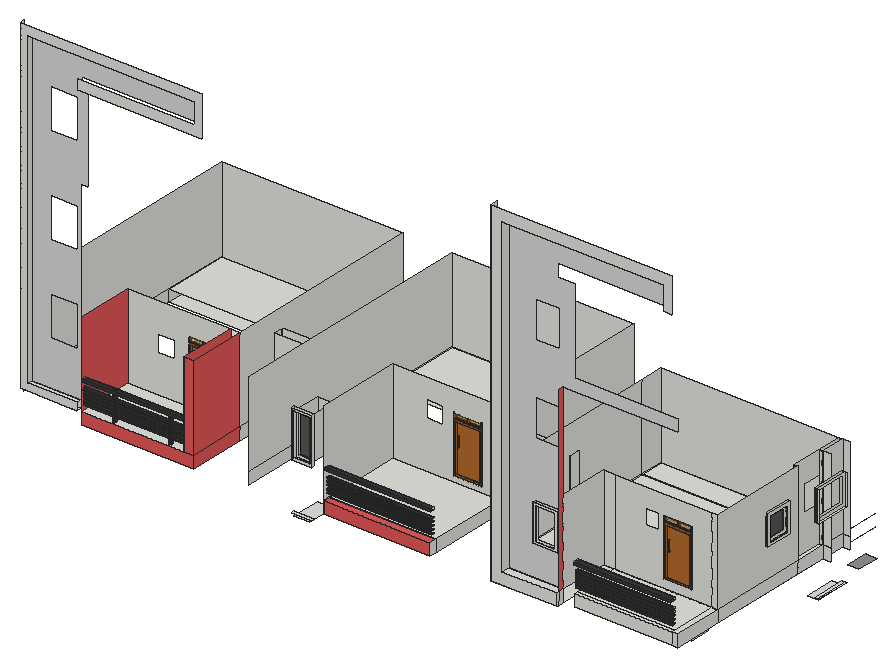
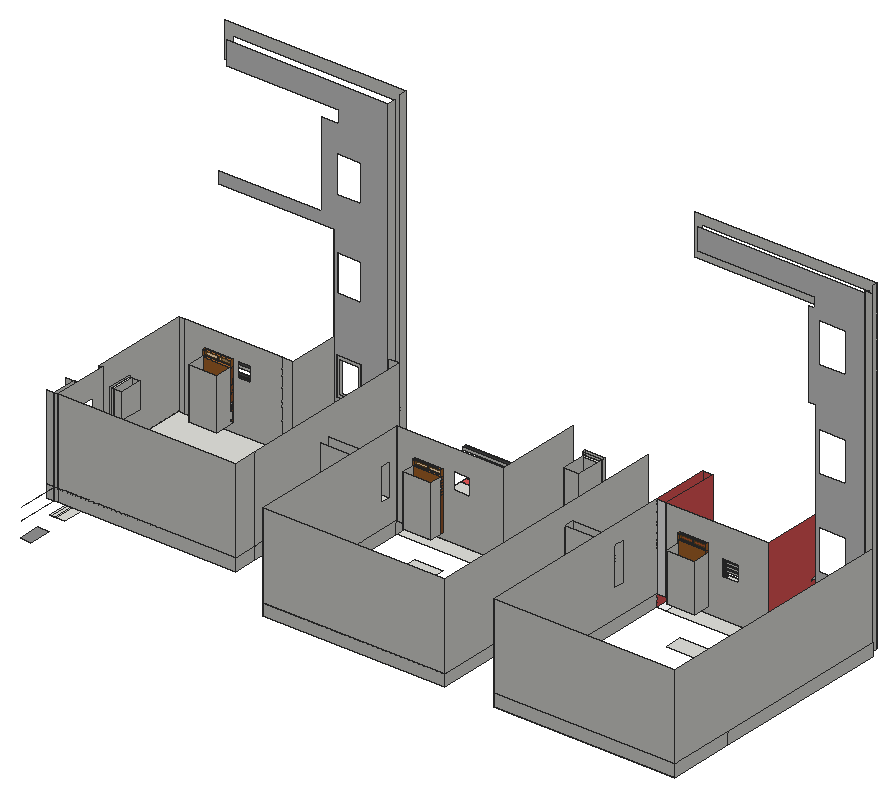
# SketchUp Ruby script. Lengths in inches.
U = 1.inch
M = Sketchup.active_model
def pt(a) = Geom::Point3d.new(a.map { |v| v * U })
def face(e, loops, mat)
  f = e.add_face(loops[0].map { |a| pt(a) })
  loops[1..].each { |l| e.add_face(l.map { |a| pt(a) }).erase! }
  f.material = f.back_material = mat if mat
  f
end
# faces: each face lists its corners as indices into pts; further lists are holes
def faces(e, pts, list, mat = nil) = list.each { |f| face(e, (f[0].is_a?(Array) ? f : [f]).map { |l| l.map { |i| pts[i] } }, mat) }
# xy, xz, yz: faces in a plane at the given z, y or x. An outline is a flat list of corners, or four numbers for a rectangle; further outlines are holes
def ring(l) = l.size == 4 ? [[l[0], l[1]], [l[2], l[1]], [l[2], l[3]], [l[0], l[3]]] : l.each_slice(2).to_a
def flat(e, list, mat, &to3) = list.each { |f| face(e, (f[0].is_a?(Array) ? f : [f]).map { |l| ring(l).map { |u, v| to3.(u, v) } }, mat) }
def xy(e, z, list, mat = nil) = flat(e, list, mat) { |x, y| [x, y, z] }
def xz(e, y, list, mat = nil) = flat(e, list, mat) { |x, z| [x, y, z] }
def yz(e, x, list, mat = nil) = flat(e, list, mat) { |y, z| [x, y, z] }
def lines(e, pts, list) = list.each { |a, b| e.add_line(pt(pts[a]), pt(pts[b])) }
# prism: a flat outline (further loops are holes) pulled along v
def prism(e, loops, v, mat = nil)
  f = face(e, loops, mat); d = Geom::Vector3d.new(v.map { |x| x * U })
  f.pushpull(f.normal.samedirection?(d) ? d.length : -d.length)
end
def box(e, o, s, mat = nil) = prism(e, [[o, [o[0] + s[0], o[1], o[2]], [o[0] + s[0], o[1] + s[1], o[2]], [o[0], o[1] + s[1], o[2]]]], [0, 0, s[2]], mat)
def at(x, y, z, deg = 0) = Geom::Transformation.translation(pt([x, y, z])) * Geom::Transformation.rotation(ORIGIN, Z_AXIS, deg.degrees)
def axes(o, x, y, z) = Geom::Transformation.new([*x, 0, *y, 0, *z, 0, *pt(o).to_a, 1])
def part(name) = M.definitions.add(name)
# library, detail: a bought-in or finely detailed component or shape, given as its bounding box
def library(name, o, s) = part(name).tap { |d| box(d.entities, o, s) }
def detail(e, o, s) = box(e.add_group.entities, o, s)
def put(e, d, t, mat = nil) = e.add_instance(d, t).tap { |i| i.material = mat if mat }
def group(e, t, mat = nil) = e.add_group.tap { |g| g.transformation = t; g.material = mat if mat }.entities
root = M.entities
M.materials.add("Generic").color = [145, 145, 145]
M.materials.add("Generic\#2").color = [229, 87, 87]
M.materials.add("Generic\#3").color = [216, 216, 216]
M.materials.add("[Color M00]").color = [255, 255, 255]
M.materials.add("[Color M07]").color = [58, 58, 58]
M.materials.add("[Color M08]").color = [45, 45, 45]
M.materials.add("[Translucent Glass Dark Green]").color = [168, 100, 12]
M.materials["[Translucent Glass Dark Green]"].alpha = 0.5
M.materials.add("[Translucent Glass Gray]").color = [0, 0, 0]
M.materials["[Translucent Glass Gray]"].alpha = 0.62
M.materials.add("[Wood Bamboo]").color = [177, 105, 43]
M.materials.add("[Wood Cherry Original]").color = [152, 86, 42]
c1 = part("Group\#10")
xy(c1.entities,0,[[0,1.08,55.8125,6.01]],"[Wood Cherry Original]")
xy(c1.entities,3.96,[[3.96,1.08,51.86,3.01]],"[Wood Bamboo]")
xy(c1.entities,51.66,[[8.63,0,9.88,3.01]],"[Color M08]")
xy(c1.entities,52.54,[[8.63,0.6875,9.88,3.01]],"[Color M08]")
xy(c1.entities,71.82,[[8.63,0.6875,9.88,3.01]],"[Color M08]")
xy(c1.entities,72.69,[[8.63,0,9.88,3.01]],"[Color M08]")
xy(c1.entities,97.36,[[3.96,1.08,51.86,3.01]],"[Wood Bamboo]")
xy(c1.entities,101.3125,[[0,1.08,55.8125,6.01]],"[Wood Bamboo]")
xy(c1.entities,102.55,[[1.23,1.08,27.29,3.01],[27.29,1.08,28.52,1.95],[28.52,1.08,54.58,3.01]],"[Wood Bamboo]")
xy(c1.entities,112.31,[[1.23,1.08,1.23,3.01,27.29,3.01,27.29,1.95,28.52,1.95,28.52,3.01,54.58,3.01,54.58,1.08]],"[Wood Bamboo]")
xy(c1.entities,113.54,[[0,1.08,55.8125,6.01]],"[Wood Bamboo]")
xz(c1.entities,0,[[8.63,51.66,9.88,72.69]],"[Color M08]")
xz(c1.entities,0.6875,[[8.63,52.54,9.88,71.82]])
xz(c1.entities,1.08,[[0,101.3125,55.8125,102.55],[0,102.55,1.23,102.55,1.23,112.31,54.58,112.31,54.58,102.55,55.8125,102.55,55.8125,113.54,0,113.54]],"[Wood Bamboo]")
xz(c1.entities,1.08,[[[0,0,55.8125,101.3125],[3.96,3.96,51.86,97.36]]],"[Wood Cherry Original]")
xz(c1.entities,1.95,[[27.29,102.55,28.52,112.31]],"[Wood Bamboo]")
xz(c1.entities,3.01,[[8.63,71.82,9.88,72.69]])
xz(c1.entities,3.01,[[1.23,102.55,27.29,112.31],[28.52,102.55,54.58,112.31]],"[Translucent Glass Dark Green]")
xz(c1.entities,3.01,[[[3.96,3.96,51.86,97.36],[8.63,71.82,9.88,72.69],[8.63,51.66,9.88,52.54]]],"[Wood Bamboo]")
xz(c1.entities,6.01,[[0,0,55.8125,101.3125],[0,112.31,55.8125,113.54]],"[Wood Bamboo]")
yz(c1.entities,0,[[1.08,101.3125,6.01,113.54]],"[Wood Bamboo]")
yz(c1.entities,0,[[1.08,0,6.01,101.3125]],"[Wood Cherry Original]")
yz(c1.entities,1.23,[[1.08,102.55,3.01,112.31]],"[Wood Bamboo]")
yz(c1.entities,3.96,[[1.08,3.96,3.01,97.36]],"[Wood Bamboo]")
yz(c1.entities,8.63,[[0,51.66,0,72.69,3.01,72.69,3.01,71.82,0.6875,71.82,0.6875,52.54,3.01,52.54,3.01,51.66]],"[Color M08]")
yz(c1.entities,9.88,[[0,51.66,3.01,51.66,3.01,52.54,0.6875,52.54,0.6875,71.82,3.01,71.82,3.01,72.69,0,72.69]],"[Color M08]")
yz(c1.entities,27.29,[[1.95,102.55,3.01,112.31]],"[Wood Bamboo]")
yz(c1.entities,28.52,[[1.95,102.55,3.01,112.31]],"[Wood Bamboo]")
yz(c1.entities,51.86,[[1.08,3.96,3.01,97.36]],"[Wood Bamboo]")
yz(c1.entities,54.58,[[1.08,102.55,3.01,112.31]],"[Wood Bamboo]")
yz(c1.entities,55.8125,[[1.08,101.3125,6.01,113.54]],"[Wood Bamboo]")
yz(c1.entities,55.8125,[[1.08,0,6.01,101.3125]],"[Wood Cherry Original]")
p = [[1.23,3.01,112.31],[1.23,6.01,112.31],[9.24,3.01,71.99],[9.24,0.51,71.99],[9.24,0.51,52.37],[9.24,3.01,52.37]]
lines(c1.entities,p,[[0,1],[2,3],[3,4],[4,5]])
c2 = part("Group\#3")
xy(c2.entities,0,[[0,0,31.25,5.5]])
xy(c2.entities,4.35,[[4.35,0,26.9,2.5]])
xy(c2.entities,79.53,[[4.35,0,26.9,2.5]])
xy(c2.entities,83.875,[[0,0,31.25,5.5]])
xz(c2.entities,0,[[[0,0,31.25,83.875],[4.35,4.35,26.9,79.53]]])
xz(c2.entities,2.5,[[4.35,4.35,26.9,79.53]],"[Translucent Glass Gray]")
xz(c2.entities,5.5,[[0,0,31.25,83.875]])
yz(c2.entities,0,[[0,0,5.5,83.875]])
yz(c2.entities,4.35,[[0,4.35,2.5,79.53]])
yz(c2.entities,26.9,[[0,4.35,2.5,79.53]])
yz(c2.entities,31.25,[[0,0,5.5,83.875]])
c3 = part("Group\#6")
xy(c3.entities,0,[[0,0,6,44.5]])
xy(c3.entities,4.57,[[3,4.57,6,39.93]])
xy(c3.entities,45.43,[[3,4.57,6,39.93]])
xy(c3.entities,50,[[0,0,6,44.5]])
xz(c3.entities,0,[[0,0,6,50]])
xz(c3.entities,4.57,[[3,4.57,6,45.43]])
xz(c3.entities,39.93,[[3,4.57,6,45.43]])
xz(c3.entities,44.5,[[0,0,6,50]])
yz(c3.entities,0,[[0,0,44.5,50]])
yz(c3.entities,3,[[4.57,4.57,39.93,45.43]],"[Translucent Glass Gray]")
yz(c3.entities,6,[[[0,0,44.5,50],[4.57,4.57,39.93,45.43]]])
xy(root,503.36,[[1435.83,421.57,1452.58,481],[1452.58,421.57,1457.58,481]])
xy(root,507.77,[[1452.58,417.16,1457.58,485.41],[1457.58,417.16,1462.21,485.41]])
xy(root,508.37,[[1429.21,528.77,1451.02,572.96]],"Generic")
xy(root,512.73,[[392.26,187.125,448.07,220.9375]])
xy(root,514.29,[[1294.76,194.1875,1315.01,199.25],[1294.76,199.25,1315.01,212.4375]])
xy(root,516.9,[[1327.46,199.25,1383.27,240]])
xy(root,517.05,[[1292.01,194.1875,1317.77,199.25]])
xy(root,519.27,[[862.05,258.8125,917.86,288.3125]])
xy(root,522.04,[[676.72,93.8125,707.97,99.8125],[676.72,99.8125,707.97,152.375]])
xy(root,526.41,[[672.35,93.8125,712.33,99.8125]])
xy(root,552,[[272.78,71.5,475.8125,187.125],[1075.83,84.125,1207.39,99.8125],[741.96,99.8125,954.11,258.8125],[1075.83,99.8125,1075.83,459.8125,1435.83,459.8125,1435.83,199.25,1207.39,199.25,1207.39,99.8125],[1230.96,99.8125,1423.39,199.25],
  [1423.39,99.8125,1435.83,199.25],[135.5,459.8125,495.5,590.625],[594.11,459.8125,954.11,590.625]])
xy(root,552,[[741.96,86,954.11,99.8125]],"Generic\#2")
xy(root,552,[[475.8125,71.5,495.5,187.125]],"[Color M00]")
xy(root,560.8125,[[135.5,90.625,248.28,99.8125]])
xy(root,576,[[[272.78,71.5,475.8125,187.125],[333.62,76.97,335.18,80.4375],[330.87,76.97,332.43,80.4375],[445.18,76.97,446.75,79.72],[442.43,76.97,444,79.66]],[330.87,76.97,332.43,80.4375],[333.62,76.97,335.18,80.4375],[442.43,76.97,444,79.66],[445.18,76.97,446.75,79.72],
  [1098.52,84.125,1207.39,99.8125],[150.0625,90.625,248.28,99.8125],[741.96,99.8125,954.11,258.8125],[1075.83,99.8125,1075.83,459.8125,1427.83,459.8125,1427.83,398.12,1435.83,398.12,1435.83,199.25,1207.39,199.25,1207.39,99.8125],[1230.96,99.8125,1423.39,107.625],
  [1423.39,99.8125,1435.83,199.25],[1230.96,107.625,1423.39,199.25],[1427.83,398.12,1435.83,459.8125],[135.5,459.8125,495.5,590.625],[594.11,459.8125,954.11,590.625],
  [1075.83,459.8125,1427.83,507.75],[1427.83,459.8125,1435.83,507.75]])
xy(root,576,[[741.96,86,954.11,99.8125]],"Generic\#2")
xy(root,576,[[475.8125,71.5,495.5,79.5],[475.8125,79.5,495.5,187.125]],"[Color M00]")
xy(root,586.3125,[[1230.96,101.06,1423.39,106.62]],"[Color M07]")
xy(root,586.39,[[272.78,74.79,492.5625,80.4375]],"[Color M07]")
xy(root,587.12,[[862.05,258.8125,917.86,288.3125]])
xy(root,587.21,[[741.96,90.58,954.11,95.39]],"[Color M07]")
xy(root,588.74,[[392.26,187.125,448.07,220.9375]])
xy(root,589.0625,[[1230.96,101.06,1423.39,106.62]],"[Color M07]")
xy(root,589.08,[[741.96,90.58,954.11,95.39]],"[Color M07]")
xy(root,589.76,[[272.78,74.79,492.5625,80.4375]],"[Color M07]")
xy(root,592.37,[[1327.46,199.25,1383.27,240]])
xy(root,593.33,[[272.78,74.79,492.5625,80.4375]],"[Color M07]")
xy(root,593.5625,[[1230.96,101.06,1423.39,106.62]],"[Color M07]")
xy(root,593.96,[[741.96,90.58,954.11,95.39]],"[Color M07]")
xy(root,595.83,[[741.96,90.58,954.11,95.39]],"[Color M07]")
xy(root,596.3125,[[1230.96,101.06,1423.39,106.62]],"[Color M07]")
xy(root,596.7,[[272.78,74.79,492.5625,80.4375]],"[Color M07]")
xy(root,600.58,[[272.78,74.79,492.5625,80.4375]],"[Color M07]")
xy(root,600.625,[[1230.96,101.06,1423.39,106.62]],"[Color M07]")
xy(root,601.4,[[741.96,90.58,954.11,95.39]],"[Color M07]")
xy(root,603.27,[[741.96,90.58,954.11,95.39]],"[Color M07]")
xy(root,603.375,[[1230.96,101.06,1423.39,106.62]],"[Color M07]")
xy(root,603.95,[[272.78,74.79,492.5625,80.4375]],"[Color M07]")
xy(root,607.25,[[1230.96,101.06,1423.39,106.62]],"[Color M07]")
xy(root,607.26,[[272.78,74.79,492.5625,80.4375]],"[Color M07]")
xy(root,608.08,[[741.96,90.58,954.11,95.39]],"[Color M07]")
xy(root,609.96,[[741.96,90.58,954.11,95.39]],"[Color M07]")
xy(root,610,[[1230.96,101.06,1423.39,106.62]],"[Color M07]")
xy(root,610.64,[[272.78,74.79,492.5625,80.4375]],"[Color M07]")
xy(root,614.01,[[272.78,74.79,492.5625,80.4375]],"[Color M07]")
xy(root,614.37,[[1230.96,101.06,1423.39,106.62]],"[Color M07]")
xy(root,614.96,[[741.96,90.58,954.11,95.39]],"[Color M07]")
xy(root,616.83,[[741.96,90.58,954.11,95.39]],"[Color M07]")
xy(root,617.12,[[1230.96,101.06,1423.39,106.62]],"[Color M07]")
xy(root,617.39,[[272.78,74.79,492.5625,80.4375]],"[Color M07]")
xy(root,621.05,[[672.35,93.8125,712.33,99.8125]])
xy(root,624.62,[[954.11,276.94,1080.05,298.38]])
xy(root,625.42,[[676.72,93.8125,707.97,99.8125],[676.72,99.8125,707.97,152.375]])
xy(root,628.82,[[442.43,76.97,444,79.66],[445.18,76.97,446.75,79.72]])
xy(root,629.01,[[272.78,72.41,492.5625,80.4375]],"[Color M07]")
xy(root,629.37,[[1230.96,96.68,1423.39,106.62]],"[Color M07]")
xy(root,629.96,[[741.96,87.45,954.11,95.39]],"[Color M07]")
xy(root,632.07,[[330.87,76.97,332.43,80.4375],[333.62,76.97,335.18,80.4375]])
xy(root,632.4375,[[495.5,271.33,593.5,290.83]])
xy(root,633.95,[[272.78,72.41,492.5625,80.4375]],"[Color M07]")
xy(root,634.31,[[1230.96,96.68,1423.39,106.62]],"[Color M07]")
xy(root,635.4,[[741.96,87.45,954.11,95.39]],"[Color M07]")
xy(root,636.27,[[1435.83,318.51,1439.83,371.82]])
xy(root,640.67,[[1414.21,322.92,1435.83,367.42],[1435.83,322.92,1439.83,367.42]])
xy(root,640.76,[[1151.9,93.8125,1200.57,99.8125]])
xy(root,642.84,[[1452.58,417.16,1457.58,485.41],[1457.58,417.16,1462.21,485.41]])
xz(root,71.5,[[272.78,552,495.5,576],[475.8125,576,495.5,744]],"Generic\#2")
xz(root,72.41,[[272.78,629.01,492.5625,633.95]],"[Color M07]")
xz(root,74.79,[[272.78,586.39,492.5625,589.76],[272.78,593.33,492.5625,596.7],[272.78,600.58,492.5625,603.95],[272.78,607.26,492.5625,610.64],[272.78,614.01,492.5625,617.39]],"[Color M07]")
xz(root,76.97,[[330.87,576,332.43,632.07],[333.62,576,335.18,632.07],[442.43,576,444,628.82],[445.18,576,446.75,628.82]],"[Color M07]")
xz(root,79.66,[[442.43,576,444,628.82]])
xz(root,79.72,[[445.18,576,446.75,628.82]])
xz(root,80.4375,[[272.78,586.39,330.87,589.76],[330.87,586.39,332.43,589.76],[332.43,586.39,333.62,589.76],[333.62,586.39,335.18,589.76],[335.18,586.39,492.5625,589.76],
  [330.87,589.76,332.43,593.33],[333.62,589.76,335.18,593.33],[272.78,593.33,330.87,596.7],[330.87,593.33,332.43,596.7],[332.43,593.33,333.62,596.7],
  [333.62,593.33,335.18,596.7],[335.18,593.33,492.5625,596.7],[330.87,596.7,332.43,600.58],[333.62,596.7,335.18,600.58],[272.78,600.58,330.87,603.95],
  [330.87,600.58,332.43,603.95],[332.43,600.58,333.62,603.95],[333.62,600.58,335.18,603.95],[335.18,600.58,492.5625,603.95],[330.87,603.95,332.43,607.26],
  [333.62,603.95,335.18,607.26],[272.78,607.26,330.87,610.64],[330.87,607.26,332.43,610.64],[332.43,607.26,333.62,610.64],[333.62,607.26,335.18,610.64],
  [335.18,607.26,492.5625,610.64],[330.87,610.64,332.43,614.01],[333.62,610.64,335.18,614.01],[272.78,614.01,330.87,617.39],[330.87,614.01,332.43,617.39],
  [332.43,614.01,333.62,617.39],[333.62,614.01,335.18,617.39],[335.18,614.01,492.5625,617.39],[330.87,617.39,332.43,629.01],[333.62,617.39,335.18,629.01],
  [272.78,629.01,330.87,633.95],[330.87,629.01,332.43,632.07],[332.43,629.01,333.62,633.95],[333.62,629.01,335.18,632.07],[335.18,629.01,492.5625,633.95],
  [330.87,632.07,332.43,633.95],[333.62,632.07,335.18,633.95]])
xz(root,84.125,[[1075.83,552,1207.39,552,1207.39,576,1098.52,576,1098.52,1198.4375,1420.08,1198.4375,1420.08,1152,1435.83,1152,1435.83,1221,1075.83,1221]])
xz(root,86,[[741.96,552,954.11,576]],"Generic\#2")
xz(root,87.45,[[741.96,629.96,954.11,635.4]],"[Color M07]")
xz(root,90.58,[[741.96,587.21,954.11,589.08],[741.96,593.96,954.11,595.83],[741.96,601.4,954.11,603.27],[741.96,608.08,954.11,609.96],[741.96,614.96,954.11,616.83]],"[Color M07]")
xz(root,90.625,[[135.5,560.8125,248.28,560.8125,248.28,576,150.0625,576,150.0625,1193.875,483.3125,1193.875,483.3125,1152,250.57,1152,250.57,1132.1875,495.5,1132.1875,495.5,1212.3125,135.5,1212.3125]])
xz(root,93.8125,[[[672.35,621.05,712.33,713.66],[676.72,625.42,707.97,709.29]],[[1151.9,640.76,1200.57,714.12],[1156.27,645.13,1196.2,709.75]]])
xz(root,95.39,[[741.96,587.21,954.11,589.08],[741.96,593.96,954.11,595.83],[741.96,601.4,954.11,603.27],[741.96,608.08,954.11,609.96],[741.96,614.96,954.11,616.83],
  [741.96,629.96,954.11,635.4]])
xz(root,96.68,[[1230.96,629.37,1423.39,634.31]],"[Color M07]")
xz(root,99.8125,[[741.96,552,954.11,576],[1075.83,552,1207.39,576],[1230.96,552,1423.39,576],[1423.39,552,1435.83,576],[135.5,560.8125,248.28,576],
  [135.5,576,150.0625,1198.3125],[1075.83,576,1098.52,744],[[672.35,621.05,712.33,713.66],[676.72,625.42,707.97,709.29]],[[1151.9,640.76,1200.57,714.12],[1156.27,645.13,1196.2,709.75]]])
xz(root,99.8125,[[[150.0625,576,248.28,576,248.28,960,263.03,960,263.03,1132.1875,250.57,1132.1875,250.57,1152,483.3125,1152,483.3125,1193.875,150.0625,1193.875],[188.42,665.13,242.3125,744.27],[188.42,840.32,242.3125,919.45],[188.42,1034.32,242.3125,1113.45]],[[1098.52,576,1207.39,576,1207.39,936,1435.83,936,1435.83,960,1230.96,960,1230.96,1128,1195.78,1128,1195.78,1152,1420.08,1152,1420.08,1198.4375,1098.52,1198.4375],[1151.9,1000.39,1200.57,1073.74],[1151.9,824.89,1200.57,898.24],[1151.9,640.76,1200.57,714.12]]],"Generic\#3")
xz(root,101.06,[[1230.96,586.3125,1423.39,589.0625],[1230.96,593.5625,1423.39,596.3125],[1230.96,600.625,1423.39,603.375],[1230.96,607.25,1423.39,610],[1230.96,614.37,1423.39,617.12]],"[Color M07]")
xz(root,106.62,[[1230.96,586.3125,1423.39,589.0625],[1230.96,593.5625,1423.39,596.3125],[1230.96,600.625,1423.39,603.375],[1230.96,607.25,1423.39,610],[1230.96,614.37,1423.39,617.12],
  [1230.96,629.37,1423.39,634.31]])
xz(root,152.375,[[676.72,625.42,707.97,709.29]])
xz(root,187.125,[[[272.78,576,475.8125,744],[392.26,588.74,448.07,702.28],[331.98,651.38,365.3125,684.7]]])
xz(root,187.125,[[475.8125,576,495.5,744]],"[Color M00]")
xz(root,199.25,[[1207.39,576,1230.96,744],[[1230.96,576,1423.39,744],[1327.46,592.37,1383.27,706.34],[1292.01,676.47,1317.77,706.8]],[1423.39,576,1435.83,744]])
xz(root,220.9375,[[392.26,588.74,448.07,683.84]])
xz(root,240,[[1327.46,501.62,1383.27,516.9],[1327.46,592.37,1383.27,693.68]])
xz(root,258.8125,[[[741.96,576,954.11,744],[862.05,587.12,917.86,699.22],[808.05,670.4,841.375,703.73]]])
xz(root,271.33,[[495.5,632.4375,593.5,707.1875]])
xz(root,276.94,[[954.11,624.62,1080.05,689.99]])
xz(root,288.3125,[[862.05,587.12,917.86,688.43]])
xz(root,290.83,[[495.5,632.4375,593.5,707.1875]])
xz(root,298.38,[[954.11,624.62,1080.05,689.99]])
xz(root,318.51,[[1435.83,636.27,1439.83,695.08]])
xz(root,322.92,[[1414.21,640.67,1435.83,690.67],[1435.83,640.67,1439.83,690.67]])
xz(root,367.42,[[1414.21,640.67,1435.83,690.67],[1435.83,640.67,1439.83,690.67]])
xz(root,371.82,[[1435.83,636.27,1439.83,695.08]])
xz(root,398.12,[[1427.83,576,1435.83,744]])
xz(root,417.16,[[1452.58,642.84,1457.58,703.27],[1457.58,642.84,1462.21,703.27]])
xz(root,459.8125,[[1075.83,552,1429.21,576],[1429.21,552,1433.58,576],[1433.58,552,1435.83,576],[1435.83,552,1451.02,576],[1429.21,576,1433.58,744],
  [1433.58,576,1435.83,744],[1435.83,576,1451.02,744]])
xz(root,485.41,[[1452.58,642.84,1457.58,703.27],[1457.58,642.84,1462.21,703.27]])
xz(root,507.75,[[1075.83,552,1429.21,576],[1429.21,552,1435.83,576],[1435.83,552,1451.02,576],[1075.83,576,1427.83,744],[1427.83,576,1429.21,744],
  [1429.21,576,1435.83,744],[1435.83,576,1451.02,744]])
xz(root,590.625,[[135.5,552,495.5,576],[594.11,552,954.11,576],[135.5,576,495.5,744],[594.11,576,954.11,744]])
yz(root,135.5,[[99.8125,552,459.8125,576],[459.8125,552,590.625,576],[90.625,560.8125,99.8125,1212.3125],[99.8125,576,590.625,744]])
yz(root,150.0625,[[90.625,576,99.8125,1193.875]])
yz(root,272.78,[[74.79,586.39,80.4375,589.76],[74.79,593.33,80.4375,596.7],[74.79,600.58,80.4375,603.95],[74.79,607.26,80.4375,610.64],[74.79,614.01,80.4375,617.39],
  [72.41,629.01,80.4375,633.95]])
yz(root,272.78,[[[71.5,576,77.61,576,77.61,586.39,74.79,586.39,74.79,589.76,80.4375,589.76,80.4375,586.39,77.61,586.39,77.61,576,187.125,576,187.125,744,71.5,744],[72.41,629.01,80.4375,633.95],[74.79,593.33,80.4375,596.7],[74.79,600.58,80.4375,603.95],[74.79,607.26,80.4375,610.64],[74.79,614.01,80.4375,617.39]]],"Generic\#2")
yz(root,330.87,[[76.97,576,80.4375,632.07]],"[Color M07]")
yz(root,332.43,[[76.97,576,80.4375,632.07]],"[Color M07]")
yz(root,333.62,[[76.97,576,80.4375,632.07]],"[Color M07]")
yz(root,335.18,[[76.97,576,80.4375,632.07]],"[Color M07]")
yz(root,392.26,[[187.125,588.74,220.9375,683.84]])
yz(root,442.43,[[76.97,576,79.66,628.82]],"[Color M07]")
yz(root,444,[[76.97,576,79.66,628.82]],"[Color M07]")
yz(root,445.18,[[76.97,576,79.72,628.82]],"[Color M07]")
yz(root,446.75,[[76.97,576,79.72,628.82]],"[Color M07]")
yz(root,448.07,[[187.125,588.74,220.9375,683.84]])
yz(root,475.8125,[[71.5,576,187.125,744]],"Generic\#2")
yz(root,492.5625,[[74.79,586.39,80.4375,589.76],[74.79,593.33,80.4375,596.7],[74.79,600.58,80.4375,603.95],[74.79,607.26,80.4375,610.64],[74.79,614.01,80.4375,617.39],
  [72.41,629.01,80.4375,633.95]])
yz(root,495.5,[[187.125,552,590.625,576],[[187.125,576,590.625,744],[271.33,632.4375,290.83,707.1875]],[271.33,632.4375,290.83,707.1875]])
yz(root,495.5,[[71.5,552,187.125,576],[71.5,576,187.125,744]],"Generic\#2")
yz(root,593.5,[[271.33,632.4375,290.83,707.1875]])
yz(root,594.11,[[86,552,459.8125,576],[459.8125,552,590.625,576],[86,576,590.625,744]])
yz(root,672.35,[[93.8125,621.05,99.8125,713.66]])
yz(root,676.72,[[93.8125,625.42,99.8125,709.29],[99.8125,625.42,152.375,709.29]])
yz(root,707.97,[[93.8125,625.42,99.8125,709.29],[99.8125,625.42,152.375,709.29]])
yz(root,712.33,[[93.8125,621.05,99.8125,713.66]])
yz(root,741.96,[[86,552,99.8125,576],[[86,576,258.8125,744],[87.45,629.96,95.39,635.4],[90.58,587.21,95.39,589.08],[90.58,593.96,95.39,595.83],[90.58,601.4,95.39,603.27],[90.58,608.08,95.39,609.96],[90.58,614.96,95.39,616.83]],[90.58,587.21,95.39,589.08],[90.58,593.96,95.39,595.83],[90.58,601.4,95.39,603.27],
  [90.58,608.08,95.39,609.96],[90.58,614.96,95.39,616.83],[87.45,629.96,95.39,635.4]])
yz(root,862.05,[[258.8125,587.12,288.3125,688.43]])
yz(root,917.86,[[258.8125,587.12,288.3125,688.43]])
yz(root,954.11,[[86,552,99.8125,576],[99.8125,552,260.5,576],[260.5,552,590.625,576],[258.8125,576,260.5,744],[[260.5,576,590.625,744],[276.94,624.62,298.38,689.99]]])
yz(root,1075.83,[[84.125,552,99.8125,576],[99.8125,552,459.8125,576],[459.8125,552,507.75,576],[84.125,576,99.8125,1221],[99.8125,576,459.8125,744],
  [459.8125,576,507.75,744]])
yz(root,1080.05,[[276.94,624.62,298.38,689.99]])
yz(root,1098.52,[[84.125,576,99.8125,1198.4375]])
yz(root,1151.9,[[93.8125,640.76,99.8125,714.12]])
yz(root,1200.57,[[93.8125,640.76,99.8125,714.12]])
yz(root,1207.39,[[84.125,552,88,576],[88,552,99.8125,576],[99.8125,576,199.25,744]])
yz(root,1207.39,[[88,576,99.8125,936]],"Generic\#2")
yz(root,1230.96,[[101.06,586.3125,106.62,589.0625],[101.06,593.5625,106.62,596.3125],[101.06,600.625,106.62,603.375],[101.06,607.25,106.62,610],[101.06,614.37,106.62,617.12],
  [96.68,629.37,106.62,634.31]])
yz(root,1327.46,[[199.25,501.62,240,516.9],[199.25,592.37,240,693.68]])
yz(root,1383.27,[[199.25,501.62,240,516.9],[199.25,592.37,240,693.68]])
yz(root,1414.21,[[322.92,640.67,367.42,690.67]])
yz(root,1427.83,[[[398.12,576,507.75,744],[421.57,647.24,481,698.86]]])
yz(root,1435.83,[[99.8125,552,199.25,576],[199.25,552,398.12,576],[398.12,552,459.8125,576],[459.8125,552,507.75,576],[[199.25,576,398.12,744],[318.51,636.27,371.82,695.08]],
  [459.8125,576,507.75,744],[[318.51,636.27,371.82,695.08],[322.92,640.67,367.42,690.67]]])
yz(root,1439.83,[[[318.51,636.27,371.82,695.08],[322.92,640.67,367.42,690.67]]])
yz(root,1452.58,[[[417.16,642.84,485.41,703.27],[421.57,647.24,481,698.86]]])
yz(root,1457.58,[[[417.16,642.84,485.41,703.27],[421.57,647.24,481,698.86]]])
p = [[272.78,77.5,588],[475.8125,77.5,588],[272.78,77.5,595],[475.8125,77.5,595],[272.78,77.5,602],[475.8125,77.5,602],
  [272.78,77.5,609],[475.8125,77.5,609],[272.78,77.5,616],[475.8125,77.5,616],[272.78,77.5,631],[475.8125,77.5,631],
  [447.03,77.61,586.39],[447.03,77.61,576],[446.75,79.72,628.82],[446.75,79.72,633.95],[445.18,79.72,628.82],[445.18,79.72,633.95],
  [445.18,76.97,628.82],[445.18,76.97,633.95],[444,76.97,628.82],[444,76.97,633.95],[442.43,76.97,628.82],[442.43,76.97,633.95],
  [444,79.66,628.82],[444,79.66,633.95],[442.43,79.66,628.82],[442.43,79.66,633.95],[450.17,78.01,632.43],[450.17,78.01,633.95],
  [442.73,76.97,632.43],[330.87,76.97,632.07],[330.87,76.97,633.95],[335.18,76.97,632.07],[335.18,76.97,633.95],[333.62,76.97,632.07],
  [333.62,76.97,633.95],[1435.83,507.75,552],[1435.83,590.625,552],[741.96,92.91,588],[954.11,92.91,588],[741.96,92.91,595],
  [954.11,92.91,595],[741.96,92.91,602],[954.11,92.91,602],[741.96,92.91,609],[954.11,92.91,609],[741.96,92.91,616],
  [954.11,92.91,616],[741.96,92.91,631],[954.11,92.91,631],[1230.96,103.72,588],[1423.39,103.72,588],[1230.96,103.72,595],
  [1423.39,103.72,595],[1230.96,103.72,602],[1423.39,103.72,602],[1230.96,103.72,609],[1423.39,103.72,609],[1230.96,103.72,616],
  [1423.39,103.72,616],[1230.96,103.72,631],[1423.39,103.72,631],[1295.23,199.25,510.08],[1295.17,199.25,510.08],[1435.83,507.75,576],
  [1435.83,590.625,576]]
lines(root,p,[[0,1],[2,3],[4,5],[6,7],[8,9],[10,11],[12,13],[14,15],[16,17],[18,19],[20,21],[22,23],
  [24,25],[26,27],[28,29],[30,28],[31,32],[33,34],[35,36],[37,38],[39,40],[41,42],[43,44],[45,46],
  [47,48],[49,50],[51,52],[53,54],[55,56],[57,58],[59,60],[61,62],[63,64],[65,66]])
put(root,c1,at(862.05,257.74,587.12))
put(root,c1,at(392.26,187.125,588.74))
put(root,c1,at(1327.46,198.1875,592.37))
put(root,c2,at(676.72,99.8125,625.42))
put(root,c3,at(1429.83,322.92,640.67))
